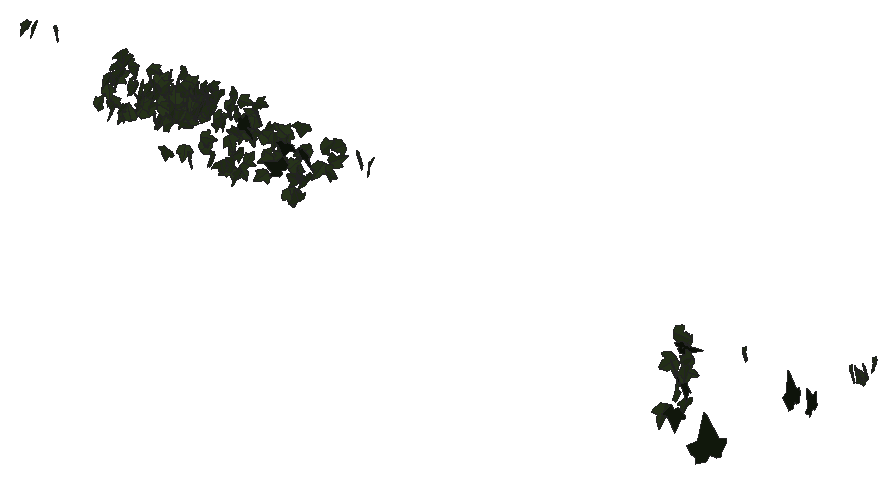
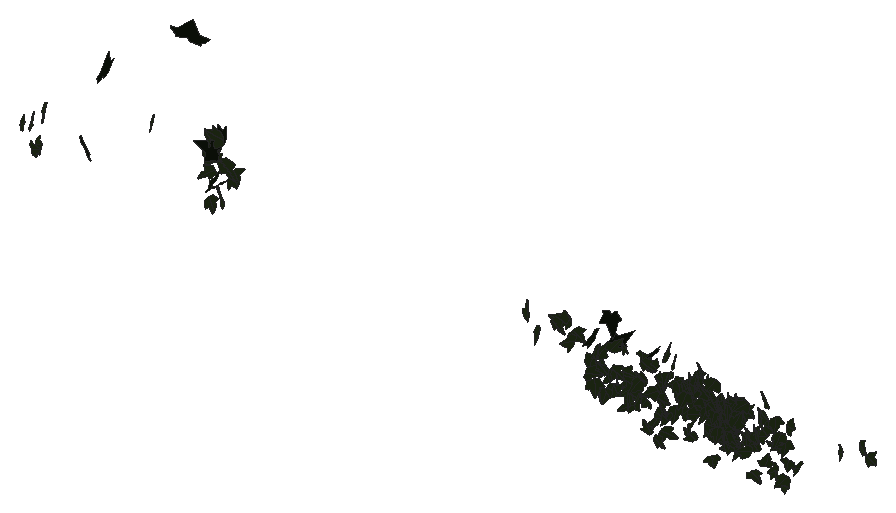
# SketchUp Ruby script. Lengths in inches.
U = 1.inch
M = Sketchup.active_model
def pt(a) = Geom::Point3d.new(a.map { |v| v * U })
def face(e, loops, mat)
  f = e.add_face(loops[0].map { |a| pt(a) })
  loops[1..].each { |l| e.add_face(l.map { |a| pt(a) }).erase! }
  f.material = f.back_material = mat if mat
  f
end
# faces: each face lists its corners as indices into pts; further lists are holes
def faces(e, pts, list, mat = nil) = list.each { |f| face(e, (f[0].is_a?(Array) ? f : [f]).map { |l| l.map { |i| pts[i] } }, mat) }
# xy, xz, yz: faces in a plane at the given z, y or x. An outline is a flat list of corners, or four numbers for a rectangle; further outlines are holes
def ring(l) = l.size == 4 ? [[l[0], l[1]], [l[2], l[1]], [l[2], l[3]], [l[0], l[3]]] : l.each_slice(2).to_a
def flat(e, list, mat, &to3) = list.each { |f| face(e, (f[0].is_a?(Array) ? f : [f]).map { |l| ring(l).map { |u, v| to3.(u, v) } }, mat) }
def xy(e, z, list, mat = nil) = flat(e, list, mat) { |x, y| [x, y, z] }
def xz(e, y, list, mat = nil) = flat(e, list, mat) { |x, z| [x, y, z] }
def yz(e, x, list, mat = nil) = flat(e, list, mat) { |y, z| [x, y, z] }
def lines(e, pts, list) = list.each { |a, b| e.add_line(pt(pts[a]), pt(pts[b])) }
# prism: a flat outline (further loops are holes) pulled along v
def prism(e, loops, v, mat = nil)
  f = face(e, loops, mat); d = Geom::Vector3d.new(v.map { |x| x * U })
  f.pushpull(f.normal.samedirection?(d) ? d.length : -d.length)
end
def box(e, o, s, mat = nil) = prism(e, [[o, [o[0] + s[0], o[1], o[2]], [o[0] + s[0], o[1] + s[1], o[2]], [o[0], o[1] + s[1], o[2]]]], [0, 0, s[2]], mat)
def at(x, y, z, deg = 0) = Geom::Transformation.translation(pt([x, y, z])) * Geom::Transformation.rotation(ORIGIN, Z_AXIS, deg.degrees)
def axes(o, x, y, z) = Geom::Transformation.new([*x, 0, *y, 0, *z, 0, *pt(o).to_a, 1])
def part(name) = M.definitions.add(name)
# library, detail: a bought-in or finely detailed component or shape, given as its bounding box
def library(name, o, s) = part(name).tap { |d| box(d.entities, o, s) }
def detail(e, o, s) = box(e.add_group.entities, o, s)
def put(e, d, t, mat = nil) = e.add_instance(d, t).tap { |i| i.material = mat if mat }
def group(e, t, mat = nil) = e.add_group.tap { |g| g.transformation = t; g.material = mat if mat }.entities
root = M.entities
M.materials.add("efeu1").color = [18, 25, 13]
M.materials.add("efeu2").color = [43, 57, 29]
c1 = part("ivyleaf_10")
p = [[0,0.5,-0.03],[-0.0625,2.02,-0.43],[-0.19,2.01,-0.46],[-0.54,1.05,-0.29],[-0.52,0.625,-0.18],[-0.83,0.76,-0.28],
  [-1.16,0.64,-0.33],[-1.15,0.33,-0.24],[-0.77,-0.39,0.02],[-0.3,-0.51,0.16],[0.04,-0.48,0.23],[-0.02,2.01,-0.4375],
  [-0.06,2.01,-0.43],[0.04,-0.49,0.23],[0.67,-0.49,0.14],[1.38,0.36,-0.2],[1.375,0.51,-0.24],[0.81,0.65,-0.19],
  [0.62,0.59,-0.15],[0.6,1.09,-0.28],[0.5,1.23,-0.31]]
faces(c1.entities,p,[[0,1,2,3,4,5,6,7,8,9,10],[11,12,0,13,14,15,16,17,18,19,20]],"efeu2")
c2 = part("ivyleaf_9")
p = [[1.54,2.16,1.25],[1.36,2.04,1.19],[-0.21,0.99,0.68],[-0.71,1.11,0.82],[-0.85,0.86,0.67],[-0.8,0.17,0.21],
  [-0.9,-0.01,0.1],[-0.67,-0.16,-0.02],[-0.08,-0.08,-0.05],[-0.03,-0.6,-0.4],[0.65,-0.88,-0.66],[0.83,-0.6,-0.49],
  [1.29,-0.42,-0.43],[1.8125,-0.07,-0.26],[1.21,0.44,0.15]]
faces(c2.entities,p,[[0,1,2,3,4,5,6,7,8,9,10,11,12,13,14]],"efeu1")
put(root,c1,axes([514.96,137.95,140.96],[0.44993,0.44593,-0.07956],[-0.06166,-0.0508,-0.63343],[-0.44876,0.45408,0.00727]))
put(root,c2,axes([585.94,126.03,141.69],[-0.09665,-0.85912,0.11291],[0.28342,-0.1387,-0.81278],[0.81884,-0.0534,0.29465]))
put(root,c1,axes([521.54,137.19,141.24],[0.31353,0.13446,-0.61128],[-0.58412,-0.18273,-0.33979],[-0.22483,0.66225,0.03036]))
put(root,c1,axes([585.26,128.875,141.25],[-0.1651,-0.64423,0.15719],[-0.02702,-0.15532,-0.66494],[0.66258,-0.16686,0.01205]))
put(root,c1,axes([585.43,124.97,142.1875],[-0.11361,-0.84946,0.50378],[0.33239,-0.51041,-0.78568],[0.93,0.07865,0.34235]))
put(root,c1,axes([522.88,136.99,141.875],[0.02373,0.66502,0.25191],[0.01241,0.25162,-0.66543],[-0.71102,0.02658,-0.0032]))
put(root,c1,axes([505.32,138.83,141.7],[0.1785,-0.34652,0.51419],[0.23047,-0.45965,-0.38978],[0.57563,0.29149,-0.00338]))
put(root,c1,axes([529.87,135.85,142.25],[0.56896,0.46628,0.22921],[0.17549,0.14748,-0.73561],[-0.48904,0.5954,0.0027]))
put(root,c1,axes([523.4375,135.875,142.08],[0.10227,-0.47894,0.44315],[0.10127,-0.43148,-0.48969],[0.6446,0.14377,0.00663]))
put(root,c1,axes([507.125,138,142.1],[0.52414,-0.33783,-0.14401],[-0.12256,0.07566,-0.62357],[0.34618,0.53827,-0.00273]))
put(root,c1,axes([515.34,134.72,142.29],[-0.61927,-0.10255,0.21179],[-0.20625,-0.05045,-0.62752],[0.11327,-0.65254,0.01524]))
put(root,c1,axes([584.05,128.62,141.625],[0.77319,-0.6332,0.25462],[-0.18281,0.17854,0.99915],[-0.65754,-0.79422,0.02162]))
put(root,c1,axes([508.24,139.99,142.49],[0.53296,0.16087,-0.33534],[-0.32095,-0.09718,-0.55671],[-0.18795,0.62214,-0.00025]))
put(root,c1,axes([505.09,138.91,142.5],[-0.43167,-0.18607,-0.43952],[0.40211,0.17746,-0.47006],[0.25711,-0.58993,-0.00277]))
put(root,c1,axes([522.31,138.6875,141.76],[0.57299,-0.06824,-0.29423],[0.29202,-0.03601,0.57704],[-0.07716,-0.64311,-0.00109]))
put(root,c1,axes([517.69,137.56,142.1],[0.49479,0.04999,-0.4406],[0.43911,0.03671,0.49727],[0.06176,-0.66151,-0.0057]))
put(root,c1,axes([521.73,135.25,142.88],[-0.40799,-0.54294,-0.15661],[0.09584,0.12388,-0.67914],[0.55689,-0.41909,0.00214]))
put(root,c2,axes([584.97,128.81,143.22],[0.2196,-0.64864,0.38226],[0.1241,-0.36156,-0.6848],[0.7426,0.25224,0.0014]))
put(root,c1,axes([519.5,141,142.77],[0.21983,-0.09412,-0.61048],[-0.55802,0.2476,-0.23911],[0.26487,0.59975,0.00292]))
put(root,c1,axes([507.01,137.99,142.29],[0.05062,-0.23009,0.59352],[-0.1589,0.57197,0.23529],[-0.6164,-0.16634,-0.01191]))
put(root,c1,axes([526.76,135.79,143.22],[0.45556,0.1131,-0.50583],[-0.50081,-0.07752,-0.46837],[-0.13359,0.67631,0.0309]))
put(root,c1,axes([511.71,137.92,143.0625],[-0.02053,-0.38529,-0.50905],[0.05002,0.50678,-0.38559],[0.63646,-0.05226,0.01388]))
put(root,c1,axes([518.9375,133.68,143.38],[-0.2609,0.30336,-0.57071],[0.33815,-0.46044,-0.39933],[-0.55081,-0.42636,0.02517]))
put(root,c1,axes([505.02,136.81,142.84],[0.13884,0.29865,-0.54476],[0.05914,0.54931,0.31622],[0.61843,-0.11958,0.09206]))
put(root,c1,axes([508.5,137.59,142.42],[0.50378,0.37937,0.10367],[-0.08844,-0.05488,0.63058],[0.38321,-0.5114,0.00923]))
put(root,c1,axes([520.44,135.51,142.93],[0.02744,-0.07451,0.68136],[0.36519,-0.57547,-0.07764],[0.58003,0.36584,0.01665]))
put(root,c1,axes([518.16,137.42,142.89],[-0.04851,0.4928,-0.44903],[-0.07189,0.44373,0.49474],[0.66281,0.08419,0.02079]))
put(root,c1,axes([512.82,137.7,142.96],[0.04123,0.04993,-0.655],[0.32341,0.5697,0.06379],[0.57177,-0.32583,0.01115]))
put(root,c1,axes([512.57,138.375,143.51],[-0.04025,-0.43309,0.47651],[-0.02359,-0.47613,-0.43473],[0.64348,-0.04454,0.01386]))
put(root,c1,axes([532.18,134.22,142.91],[-0.30843,-0.59557,-0.27554],[-0.12633,-0.24487,0.6707],[-0.64394,0.3333,0.00039]))
put(root,c1,axes([511.85,137.47,142.64],[-0.47471,0.42743,-0.05893],[-0.04515,0.03792,0.63878],[0.4291,0.47685,0.00202]))
put(root,c2,axes([598.58,131.88,143.8],[-0.11762,0.29479,0.87947],[-0.36555,0.80004,-0.31705],[-0.8525,-0.38373,0.01461]))
put(root,c1,axes([524.84,138.33,143.5625],[0.13178,0.19349,0.62545],[0.36399,0.50866,-0.23405],[-0.54419,0.38708,-0.00509]))
put(root,c1,axes([512.74,138.49,143.61],[0.10476,-0.05457,0.6283],[0.63066,0.00729,-0.10452],[0.00176,0.63693,0.05503]))
put(root,c1,axes([510.21,138.27,143.5],[-0.04682,-0.22264,0.63889],[0.10982,0.62942,0.22739],[-0.6676,0.11916,-0.0074]))
put(root,c1,axes([505.08,138.3,144.11],[0.60145,0.08302,0.1919],[0.19023,0.02524,-0.60716],[-0.08677,0.63082,-0.00097]))
put(root,c1,axes([509.98,137.3,143.5],[0.55484,0.10246,-0.33743],[0.33118,0.06473,0.56422],[0.12116,-0.64616,0.00302]))
put(root,c1,axes([515.32,137.54,144.36],[-0.22755,-0.44365,-0.43111],[0.24106,0.35945,-0.49714],[0.56971,-0.32929,0.03816]))
put(root,c1,axes([514.4,138.15,143.54],[-0.48708,-0.19327,0.39528],[0.3698,0.13972,0.524],[-0.23842,0.61154,0.00521]))
put(root,c1,axes([528.375,139.125,144.57],[0.37921,-0.49957,-0.29594],[-0.16753,0.2443,-0.62706],[0.55595,0.41437,0.0129]))
put(root,c1,axes([583.9,128.34,145.57],[0.72198,-0.17196,-0.7603],[-0.7243,0.23507,-0.74096],[0.28813,1.02179,0.04251]))
put(root,c1,axes([522.34,136.12,144.5],[0.39712,-0.09392,0.50944],[0.50058,-0.09561,-0.40784],[0.13331,0.63882,0.01386]))
put(root,c1,axes([585.08,128.83,144.59],[0.14853,0.26175,0.66204],[0.32677,0.57578,-0.30095],[-0.63248,0.35894,-0.00002]))
put(root,c1,axes([512.01,138.54,144.84],[-0.42802,-0.17943,0.4451],[-0.41078,-0.17138,-0.46411],[0.24813,-0.59324,-0.00055]))
put(root,c1,axes([532.22,135.44,144.49],[-0.24102,-0.46735,-0.58776],[-0.20941,-0.55097,0.52397],[-0.72113,0.31619,0.04429]))
put(root,c1,axes([512.96,138.8,144.89],[0.22219,-0.28036,-0.54057],[-0.2838,0.46143,-0.35597],[0.53877,0.35869,0.03541]))
put(root,c1,axes([523.63,135.92,144.4],[-0.03765,0.02359,-0.66136],[-0.19858,-0.63231,-0.01125],[-0.63128,0.1975,0.04298]))
put(root,c1,axes([522.57,138.71,145.03],[0.50971,-0.03187,0.45632],[0.45542,-0.02867,-0.5107],[0.04287,0.68353,-0.00014]))
put(root,c1,axes([513.54,137.52,144.94],[-0.32626,-0.54441,-0.12974],[0.07884,0.10397,-0.63453],[0.55407,-0.33536,0.01389]))
put(root,c1,axes([510.21,137.22,145.1],[0.00623,0.41985,-0.50432],[-0.06588,-0.50139,-0.41823],[-0.65289,0.0546,0.03739]))
put(root,c1,axes([511.66,138.62,145.01],[0.59925,-0.22119,-0.03341],[-0.02836,0.01964,-0.63871],[0.22189,0.59986,0.00859]))
put(root,c1,axes([524.22,139.4,145.28],[0.10888,-0.48751,-0.43349],[-0.10788,0.41998,-0.49941],[0.64338,0.15292,-0.01038]))
put(root,c1,axes([510.28,137.39,144.61],[0.38571,-0.16844,-0.486],[0.47706,-0.10996,0.41672],[-0.19231,-0.61063,0.05902]))
put(root,c1,axes([526.78,139.18,145.13],[0.21048,0.0558,-0.64674],[-0.64682,-0.03941,-0.21391],[-0.05484,0.67899,0.04074]))
put(root,c1,axes([519.34,135.6,144.84],[-0.06522,-0.04534,-0.6401],[0.63748,0.06912,-0.06985],[0.0735,-0.63969,0.03782]))
put(root,c1,axes([529.72,136.32,144.77],[0.51753,-0.03304,-0.47466],[0.47508,-0.00288,0.51819],[-0.0263,-0.70223,0.02021]))
put(root,c1,axes([528.47,136.45,145.37],[-0.32739,-0.2576,0.55576],[-0.44443,-0.33377,-0.41651],[0.42155,-0.55195,-0.0075]))
put(root,c1,axes([513.05,139.55,145.4],[-0.24005,-0.5896,-0.15276],[0.07722,0.13341,-0.63626],[0.60416,-0.25132,0.02063]))
put(root,c1,axes([514.92,137.2,145.32],[-0.4431,-0.48512,0.07064],[-0.04733,-0.05245,-0.65703],[0.48795,-0.44562,0.00042]))
put(root,c1,axes([510.03,137.96,144.71],[-0.1862,-0.46109,0.44643],[0.22127,0.39022,0.49532],[-0.60245,0.28583,0.04394]))
put(root,c1,axes([509.51,137.49,144.78],[-0.34248,-0.03574,0.5351],[0.47175,-0.32207,0.28042],[0.25509,0.54763,0.19984]))
put(root,c1,axes([527.65,135.625,145.09],[-0.14585,-0.07919,0.66045],[-0.56673,-0.33921,-0.16583],[0.34826,-0.58516,0.00675]))
put(root,c1,axes([514.8125,137.4,144.73],[0.59839,-0.1076,-0.28282],[0.28332,-0.02091,0.6074],[-0.10629,-0.66153,0.02681]))
put(root,c1,axes([521.73,137.65,145.08],[0.0551,-0.03845,-0.6607],[-0.62584,0.21262,-0.06457],[0.21526,0.62798,-0.0186]))
put(root,c1,axes([532.01,134.32,145.08],[-0.25887,-0.36082,-0.57278],[-0.32719,-0.47016,0.44405],[-0.59264,0.41718,0.00504]))
put(root,c1,axes([526.59,138.26,145.32],[0.18895,-0.11888,0.68053],[0.54585,-0.40676,-0.22261],[0.42344,0.57738,-0.01671]))
put(root,c1,axes([514.5,139.27,145.47],[0.08097,-0.34471,0.5667],[0.16038,-0.54379,-0.35369],[0.64362,0.17887,0.01684]))
put(root,c1,axes([586.1,127.29,144.77],[0.27407,0.69054,-0.14624],[0.04783,0.13835,0.74291],[0.70423,-0.27814,0.00645]))
put(root,c1,axes([506.29,138.48,145.76],[0.19491,-0.51288,0.32323],[0.15027,-0.28806,-0.54768],[0.58732,0.24391,0.03286]))
put(root,c1,axes([531.85,134.83,145.9],[-0.16542,0.66989,-0.17543],[0.04276,-0.17014,-0.69001],[-0.69116,-0.17086,-0.0007]))
put(root,c1,axes([529.78,138.78,145.68],[0.16389,0.15728,-0.66961],[-0.47018,-0.4768,-0.22707],[-0.50204,0.49789,-0.00593]))
put(root,c1,axes([515.75,137.98,145.92],[-0.09752,-0.47273,-0.46587],[0.11582,0.45153,-0.48242],[0.65353,-0.15057,0.01598]))
put(root,c1,axes([512.38,137.75,145.21],[0.459,0.11605,-0.44595],[0.35495,0.31233,0.44663],[0.29384,-0.55857,0.15709]))
put(root,c1,axes([525.92,139.23,145.13],[0.09011,0.5689,-0.35279],[0.05692,0.34817,0.57599],[0.66699,-0.10657,-0.00149]))
put(root,c1,axes([516.53,136.92,145.25],[-0.28668,-0.24816,0.55822],[0.40228,0.38737,0.3788],[-0.45974,0.4937,-0.01662]))
put(root,c1,axes([505.62,138.125,145.89],[-0.37225,-0.50574,-0.14921],[0.10247,0.10978,-0.62774],[0.51724,-0.38572,0.01698]))
put(root,c1,axes([600.6875,137.34,145.3],[0.3378,-0.03589,0.60831],[-0.60659,0.04654,0.33959],[-0.05812,-0.69425,-0.00868]))
put(root,c1,axes([514.14,137.49,145.93],[-0.53744,-0.34916,-0.13508],[0.11067,0.07759,-0.64089],[0.35764,-0.5487,-0.00466]))
put(root,c1,axes([517.27,138.36,145.27],[-0.04501,0.05779,0.66251],[-0.38702,-0.54227,0.021],[0.54081,-0.38325,0.07017]))
put(root,c1,axes([586.18,127.4,145.84],[-0.08504,-0.63344,0.00731],[0.14633,-0.02682,-0.62161],[0.61635,-0.08103,0.14859]))
put(root,c1,axes([525.01,137.91,145.97],[0.29981,0.25988,0.56262],[0.41776,0.3769,-0.39671],[-0.45776,0.51417,0.00644]))
put(root,c1,axes([511.13,139,145.96],[0.32799,-0.2916,0.48272],[0.37227,-0.30752,-0.43871],[0.42363,0.49601,0.01179]))
put(root,c1,axes([508.625,138.13,145.68],[0.06008,-0.19934,0.62727],[0.19861,-0.59503,-0.20812],[0.62751,0.20741,0.00582]))
put(root,c2,axes([586.07,125.98,146.14],[0.1487,-0.33109,0.86056],[0.30532,-0.80483,-0.36241],[0.87004,0.33902,-0.0199]))
put(root,c1,axes([522.99,134.96,146.16],[0.26759,0.63699,0.15355],[0.06062,0.14108,-0.69091],[-0.65243,0.27437,-0.00122]))
put(root,c1,axes([518.25,140.86,145.4375],[0.18224,0.44503,-0.4286],[0.14957,0.40179,0.48079],[0.59949,-0.23553,0.01033]))
put(root,c1,axes([600.55,136.8125,145.6875],[-0.19647,0.23082,-0.65359],[-0.45508,0.46947,0.30259],[0.52284,0.49536,0.01778]))
put(root,c1,axes([513.66,136.13,145.97],[0.21043,0.22263,0.61127],[0.42781,0.43665,-0.30631],[-0.4901,0.47674,-0.00491]))
put(root,c1,axes([506.18,138.59,145.62],[0.38779,0.02328,-0.51446],[0.44919,0.29969,0.35215],[0.25188,-0.5703,0.16405]))
put(root,c1,axes([522.48,140.37,145.46],[-0.38395,0.39142,-0.35892],[-0.24664,0.26082,0.54827],[0.47032,0.45631,-0.00549]))
put(root,c1,axes([527.125,139.12,146.45],[-0.02376,0.55589,-0.39749],[0.00129,-0.3977,-0.55625],[-0.68338,-0.02008,0.01277]))
put(root,c1,axes([509.53,139.0625,145.5],[0.37087,-0.43016,0.34434],[-0.21409,0.26997,0.56784],[-0.50772,-0.42806,0.01209]))
put(root,c1,axes([525.9,131.68,145.63],[-0.27385,0.5755,0.41446],[0.17148,-0.37737,0.6373],[0.68816,0.32305,0.00613]))
put(root,c1,axes([524.46,139.04,145.74],[0.0536,-0.08951,0.69254],[-0.141,0.67889,0.09866],[-0.68392,-0.14698,0.03394]))
put(root,c1,axes([527.26,141.09,146.46],[-0.63139,-0.34105,0.12031],[-0.10587,-0.05716,-0.71762],[0.34581,-0.64021,-0.00002]))
put(root,c1,axes([509.4375,137.85,145.32],[0.51162,-0.44222,0.07315],[-0.04817,0.05612,0.67616],[-0.44563,-0.51376,0.01089]))
put(root,c1,axes([519.83,137.33,145.9],[-0.07045,-0.14398,-0.63088],[-0.08664,-0.62679,0.15272],[-0.64127,0.1005,0.04867]))
put(root,c1,axes([513.98,138,146.5625],[0.26274,-0.5423,-0.26097],[-0.10739,0.23794,-0.60257],[0.59217,0.28377,0.00652]))
put(root,c1,axes([506.55,138.35,146.5],[-0.11319,-0.60518,0.21047],[-0.03776,-0.20706,-0.61567],[0.63962,-0.11932,0.0009]))
put(root,c1,axes([534.39,135.18,147.03],[0.45329,0.48758,-0.45262],[-0.33391,-0.30698,-0.66509],[-0.57542,0.56223,0.02939]))
put(root,c1,axes([514.74,136.39,145.97],[-0.19609,0.0677,0.65477],[0.40706,-0.52445,0.17612],[0.51732,0.43833,0.10961]))
put(root,c1,axes([511.52,137.68,145.8125],[0.16346,-0.59471,0.29974],[-0.07308,0.29076,0.61673],[-0.66195,-0.17895,0.00593]))
put(root,c1,axes([513.95,138.81,146.66],[0.55661,0.28952,0.18915],[0.16746,0.08794,-0.62741],[-0.30258,0.58126,0.00071]))
put(root,c1,axes([506.61,136.36,146.68],[0.10158,-0.35249,0.55094],[0.19726,-0.51507,-0.36591],[0.62359,0.22035,0.02601]))
put(root,c1,axes([513.68,138.25,146.45],[0.08358,-0.19679,0.62358],[0.20758,-0.58815,-0.21343],[0.62007,0.22342,-0.0126]))
put(root,c1,axes([586.02,128.59,146.32],[0.05966,0.02219,-0.63663],[-0.62707,0.11462,-0.05477],[0.11215,0.62906,0.03244]))
put(root,c1,axes([523.88,137.51,146.35],[0.11772,-0.05782,-0.69253],[0.61442,-0.31951,0.13112],[-0.32469,-0.62559,-0.00296]))
put(root,c1,axes([505.86,138.72,146.91],[-0.3643,-0.43342,-0.3087],[0.21915,0.21872,-0.56569],[0.4849,-0.42447,0.02373]))
put(root,c2,axes([530.73,133.32,146.16],[0.02085,0.03805,0.771],[-0.7094,-0.30316,0.03414],[0.30436,-0.70921,0.02677]))
put(root,c1,axes([513.95,137.41,147.01],[-0.59719,-0.31465,-0.15769],[0.13899,0.07448,-0.67501],[0.32334,-0.61315,-0.00107]))
put(root,c2,axes([584.63,128.76,147.08],[0.50887,0.34399,-0.60264],[0.49755,0.34003,0.61422],[0.48368,-0.71169,0.00218]))
put(root,c1,axes([518.7,141.21,146.91],[0.23228,-0.21789,-0.57506],[-0.43746,0.37348,-0.31821],[0.43219,0.49513,-0.01304]))
put(root,c1,axes([515.97,137.99,147.125],[0.50402,0.52673,-0.12343],[-0.08683,-0.08775,-0.72903],[-0.53399,0.51144,0.00204]))
put(root,c1,axes([511.3,137.03,147.09],[0.01268,-0.5141,0.4136],[0.06284,-0.41086,-0.51261],[0.65682,0.04923,0.04106]))
put(root,c1,axes([513.1,138.34,146.44],[0.43537,-0.19174,-0.44873],[0.40038,-0.20342,0.47538],[-0.27896,-0.59121,-0.01803]))
put(root,c1,axes([518.08,137.15,146.53],[0.21166,-0.02533,-0.6096],[0.60778,-0.04773,0.21301],[-0.05341,-0.64353,0.0082]))
put(root,c1,axes([514.59,138.72,147.2],[-0.15478,-0.51963,0.38028],[-0.04153,-0.38224,-0.53922],[0.64258,-0.14987,0.05675]))
put(root,c1,axes([513.59,137.07,147.36],[0.4356,-0.29002,0.50617],[0.41569,-0.2889,-0.52326],[0.40929,0.60207,-0.00726]))
put(root,c1,axes([511.22,139.08,146.56],[-0.43689,-0.33084,-0.35437],[-0.28758,-0.20719,0.54798],[-0.3903,0.523,-0.00709]))
put(root,c2,axes([531.79,135.46,147.54],[0.5345,-0.57226,0.02469],[0.021,-0.01417,-0.78303],[0.57241,0.53488,0.00567]))
put(root,c1,axes([508.84,138.1,147.42],[0.32016,-0.34602,0.48583],[0.31496,-0.37017,-0.4712],[0.50651,0.44889,-0.01409]))
put(root,c1,axes([520.25,136.42,146.93],[-0.00906,-0.01678,-0.70201],[0.44591,0.54222,-0.01871],[0.54247,-0.44598,0.00366]))
put(root,c1,axes([586.17,128.01,146.77],[-0.01602,0.10649,0.67535],[0.17192,-0.6532,0.10707],[0.66173,0.17228,-0.01146]))
put(root,c1,axes([515.4,137.63,147.59],[-0.43475,-0.05458,-0.5217],[0.51492,0.08485,-0.43797],[0.10006,-0.67378,-0.0129]))
put(root,c1,axes([518.93,136.94,147.46],[-0.32299,-0.61615,0.01228],[-0.00417,-0.01167,-0.69568],[0.61626,-0.32301,0.00173]))
put(root,c1,axes([524.16,135.66,146.89],[-0.34551,-0.18373,0.5424],[0.46975,0.2714,0.39116],[-0.32755,0.58302,-0.01116]))
put(root,c1,axes([518.32,137.55,147.75],[-0.17658,-0.59656,-0.31248],[0.07866,0.30256,-0.62207],[0.66883,-0.19309,-0.00934]))
put(root,c1,axes([521.07,137.25,147.62],[-0.35419,0.45141,0.33193],[-0.20835,0.25843,-0.57377],[-0.52014,-0.41091,0.0038]))
put(root,c1,axes([536.74,138.07,147.67],[-0.5527,0.51618,0.04112],[-0.03235,0.0256,-0.75624],[-0.5168,-0.55364,0.00336]))
put(root,c1,axes([522.46,140.08,147.75],[-0.21294,-0.35171,-0.57583],[0.26126,0.51374,-0.41041],[0.62211,-0.33614,-0.02474]))
put(root,c1,axes([520.49,140.1,147.43],[-0.21062,-0.11682,-0.592],[0.5469,0.22799,-0.23957],[0.25497,-0.58553,0.02483]))
put(root,c1,axes([517.82,137.34,146.7],[0.45817,0.44433,-0.12968],[0.08842,0.09509,0.63821],[0.45434,-0.46658,0.00658]))
put(root,c1,axes([513.55,138.69,147.67],[0.28894,-0.24192,0.60536],[0.49619,-0.34786,-0.37585],[0.42283,0.57354,0.02739]))
put(root,c2,axes([600.48,113.47,147.5625],[-1.34901,-0.13251,0.15894],[0.15923,0.00487,1.35546],[-0.13217,1.35833,0.01065]))
put(root,c1,axes([518.77,135.49,147.83],[0.03148,-0.74668,0.07871],[0.00824,-0.07843,-0.74732],[0.75077,0.03217,0.00491]))
put(root,c1,axes([516.95,139.7,147.98],[-0.28494,-0.5139,-0.37911],[0.22185,0.30962,-0.58645],[0.59883,-0.35924,0.03688]))
put(root,c1,axes([535.99,134.24,147.48],[-0.07141,0.03664,-0.75321],[0.64166,-0.3945,-0.08002],[-0.39615,-0.64559,0.00615]))
put(root,c1,axes([601.93,133.88,148.13],[-0.5055,0.51827,0.32896],[-0.23238,0.23286,-0.72396],[-0.56817,-0.55635,0.00343]))
put(root,c1,axes([512.34,136.72,147.77],[-0.58719,0.14148,0.21251],[-0.21118,0.03031,-0.6037],[-0.14346,-0.62373,0.01887]))
put(root,c1,axes([512.26,138.95,147.86],[0.10795,-0.56389,-0.28607],[-0.06674,0.27842,-0.574],[0.62877,0.12636,-0.01182]))
put(root,c1,axes([517.71,137.79,147.34],[0.00623,0.03633,-0.6792],[-0.01322,-0.67909,-0.03644],[-0.68004,0.01353,-0.00551]))
put(root,c1,axes([514.66,136.93,146.73],[0.62344,0.24269,0.04127],[-0.04786,0.00925,0.66851],[0.24148,-0.62474,0.02593]))
put(root,c1,axes([528.02,135.57,147.9375],[0.5819,-0.21823,0.28683],[0.26762,-0.10322,-0.62147],[0.2414,0.64049,-0.00243]))
put(root,c2,axes([524.27,135.7,148.44],[0.27287,-0.65451,-0.29958],[-0.10793,0.27956,-0.70908],[0.71168,0.29335,0.00732]))
put(root,c1,axes([507.03,139.26,147.83],[0.06604,-0.45119,0.46437],[0.04532,-0.46241,-0.45573],[0.64588,0.07858,-0.0155]))
put(root,c1,axes([602.0625,136.07,146.91],[-0.4583,0.52209,0.12956],[0.07796,-0.10394,0.69464],[0.53225,0.46478,0.00981]))
put(root,c1,axes([511.85,138.46,147.47],[-0.0243,0.08812,-0.63188],[-0.13863,-0.61795,-0.08085],[-0.62275,0.13413,0.04265]))
put(root,c1,axes([512.83,136.97,147.43],[0.13216,0.20273,-0.6363],[0.34382,0.53541,0.242],[0.5725,-0.36834,0.00156]))
put(root,c1,axes([532.94,137.4375,147.57],[0.03707,0.12736,-0.75036],[0.29436,0.69039,0.13172],[0.70186,-0.29627,-0.01561]))
put(root,c1,axes([521.41,137.96,147.3],[0.03422,-0.00782,0.66223],[0.64729,-0.13988,-0.0351],[0.1401,0.64819,0.00042]))
put(root,c1,axes([495.15,138.09,147.97],[-0.01113,-0.50512,0.39183],[-0.00122,-0.39187,-0.50521],[0.63928,-0.00955,0.00586]))
put(root,c1,axes([498.07,138.83,147.98],[-0.23582,0.29664,-0.51951],[0.30532,-0.42054,-0.37872],[-0.51446,-0.38556,0.01337]))
put(root,c1,axes([510.19,135.36,147.61],[0.16544,-0.26715,-0.63044],[0.47774,-0.41959,0.30317],[-0.4905,-0.49877,0.08264]))
put(root,c1,axes([518.09,138.3,147.05],[-0.06118,-0.61834,0.14257],[0.01201,0.14208,0.62136],[-0.63445,0.06232,-0.00199]))
put(root,c1,axes([512.43,137.34,148.28],[0.20738,-0.40776,-0.52662],[-0.23962,0.46895,-0.45747],[0.62144,0.3169,-0.00065]))
put(root,c1,axes([602.01,137.46,147.73],[0.073,-0.17636,0.61055],[0.38701,-0.47513,-0.18352],[0.50408,0.39032,0.05248]))
put(root,c1,axes([518.36,137.3,148.19],[-0.17982,0.35131,-0.52353],[0.22543,-0.47259,-0.39456],[-0.5888,-0.28823,0.00882]))
put(root,c1,axes([523.9,137.34,148.25],[0.37229,0.0556,-0.56665],[-0.56778,-0.01434,-0.37444],[-0.04255,0.67785,0.03856]))
put(root,c1,axes([512.25,137.25,147.71],[0.46343,0.20908,-0.50218],[0.39942,0.31707,0.50061],[0.36928,-0.60533,0.08876]))
put(root,c1,axes([517.66,138.94,147.5],[-0.41309,0.18815,0.45686],[0.42286,-0.17339,0.45375],[0.25557,0.59102,-0.01233]))
put(root,c1,axes([508.18,138.07,147.81],[0.2053,-0.1159,-0.63974],[0.54717,-0.33154,0.23565],[-0.35115,-0.58437,-0.00681]))
put(root,c1,axes([524.89,136.32,148.33],[0.70787,-0.0304,0.07421],[0.07454,0.0062,-0.70846],[0.02959,0.71172,0.00934]))
put(root,c1,axes([518.66,138.66,148.22],[-0.26436,-0.5788,0.1034],[-0.03888,-0.09591,-0.6363],[0.58668,-0.26716,0.00443]))
put(root,c1,axes([522.13,135.07,147.7],[-0.1875,0.08828,0.63772],[0.43647,-0.47084,0.19351],[0.47326,0.46921,0.07419]))
put(root,c1,axes([539.2,136.74,147.86],[0.17656,-0.54431,-0.5156],[0.15157,-0.49285,0.5722],[-0.73426,-0.23262,-0.00586]))
put(root,c1,axes([516.25,136.93,148.46],[0.42447,-0.31752,0.4452],[0.34833,-0.27744,-0.52998],[0.42153,0.549,-0.01035]))
put(root,c1,axes([515.625,136.96,148.74],[-0.53547,-0.25113,-0.44326],[0.41877,0.14926,-0.59045],[0.29014,-0.67892,0.03415]))
put(root,c1,axes([514.07,139.11,148.66],[0.39524,-0.35197,-0.48398],[-0.36573,0.31703,-0.52922],[0.47367,0.53847,-0.00477]))
put(root,c1,axes([518.96,134.96,148.37],[0.56038,-0.4294,0.00961],[0.00797,-0.00539,-0.70598],[0.42943,0.56044,0.00057]))
put(root,c2,axes([601.28,125.61,148.34],[-0.13735,-0.85431,0.62675],[0.263,0.58473,0.85467],[-1.0264,0.26415,0.13513]))
put(root,c1,axes([535.3,137.15,148.77],[0.45624,-0.13028,-0.61839],[-0.57672,0.22604,-0.47311],[0.25841,0.73448,0.03592]))
put(root,c1,axes([510.83,138.03,148.46],[-0.36083,-0.15428,-0.51251],[0.48263,0.17344,-0.392],[0.2314,-0.60232,0.01841]))
put(root,c1,axes([535.72,135.39,147.91],[-0.23359,-0.26847,0.6558],[0.42738,0.49742,0.35587],[-0.56524,0.48705,-0.00195]))
put(root,c1,axes([506.5,138.63,148.4375],[-0.26625,-0.58741,-0.11458],[0.05072,0.10281,-0.64493],[0.59633,-0.27101,0.0037]))
put(root,c2,axes([531.31,133.34,149.24],[0.45626,0.36643,-0.511],[-0.42257,-0.28885,-0.58444],[-0.46565,0.62118,0.02967]))
put(root,c1,axes([496.53,137.58,148.6],[0.28267,-0.53181,0.27789],[0.12334,-0.24912,-0.60222],[0.58722,0.30832,-0.00727]))
put(root,c1,axes([591.73,129.76,148.57],[-0.33023,0.46434,0.29219],[-0.17102,0.23692,-0.56979],[-0.52129,-0.37188,0.00183]))
put(root,c1,axes([517.17,138.35,148.6],[0.17791,-0.40227,0.52736],[0.22527,-0.4769,-0.43978],[0.62385,0.28693,0.00841]))
put(root,c1,axes([516.6,137.83,148.67],[0.29557,-0.60579,0.15281],[0.05994,-0.14077,-0.674],[0.62188,0.30149,-0.00767]))
put(root,c1,axes([515.09,138.51,148.03],[0.52972,-0.08575,-0.43916],[0.44001,-0.02382,0.53539],[-0.08129,-0.68767,0.03621]))
put(root,c1,axes([517.19,137.3,148.04],[-0.26723,-0.01678,0.64432],[0.64446,0.0039,0.26739],[-0.01003,0.69753,0.01401]))
put(root,c1,axes([585.67,128.8,147.98],[0.2942,-0.0834,0.56086],[-0.52898,0.18719,0.30531],[-0.20421,-0.60505,0.01715]))
put(root,c1,axes([517.34,137.9,148.1],[0.03983,-0.10485,0.68744],[0.69504,-0.01578,-0.04268],[0.022,0.68841,0.10373]))
put(root,c1,axes([528.48,136.71,147.98],[0.32748,0.48649,0.41572],[-0.22328,-0.35077,0.58638],[0.5997,-0.39626,-0.00869]))
put(root,c1,axes([584.3,128.68,148.54],[0.01676,-0.00273,-0.9619],[0.90178,-0.33475,0.01667],[-0.33474,-0.90193,-0.00327]))
